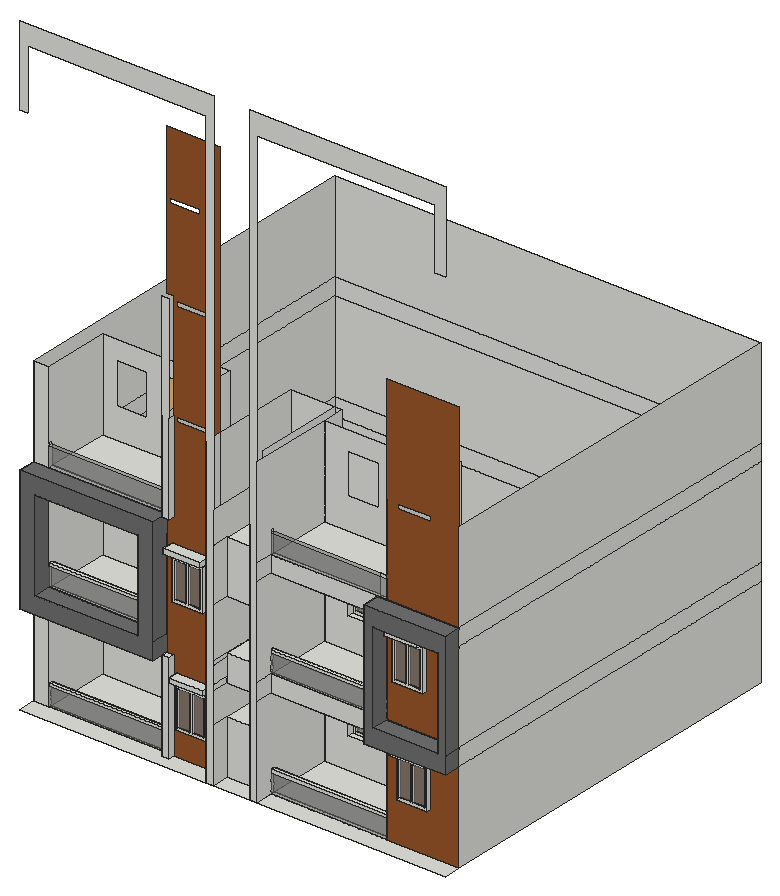
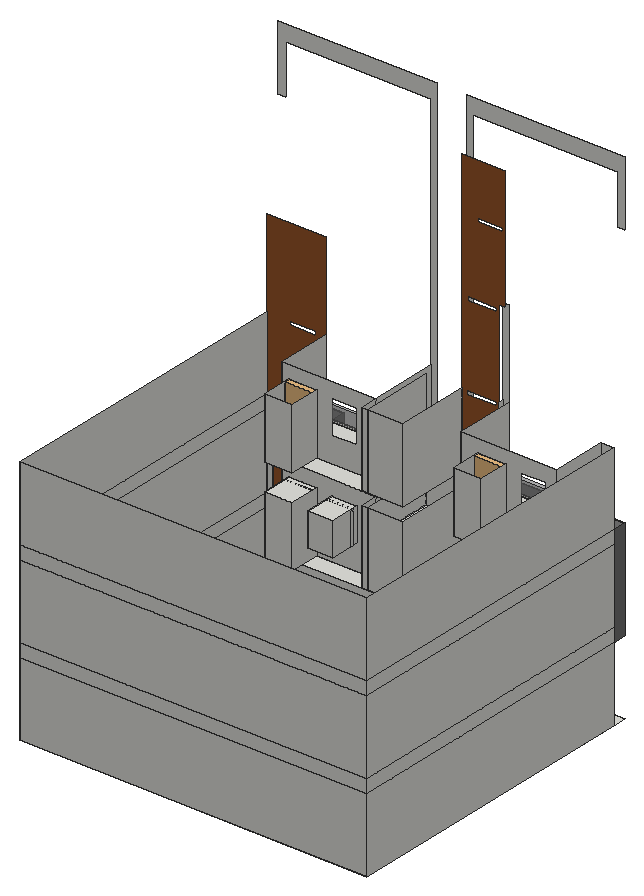
# SketchUp Ruby script. Lengths in inches.
U = 1.inch
M = Sketchup.active_model
def pt(a) = Geom::Point3d.new(a.map { |v| v * U })
def face(e, loops, mat)
  f = e.add_face(loops[0].map { |a| pt(a) })
  loops[1..].each { |l| e.add_face(l.map { |a| pt(a) }).erase! }
  f.material = f.back_material = mat if mat
  f
end
# faces: each face lists its corners as indices into pts; further lists are holes
def faces(e, pts, list, mat = nil) = list.each { |f| face(e, (f[0].is_a?(Array) ? f : [f]).map { |l| l.map { |i| pts[i] } }, mat) }
# xy, xz, yz: faces in a plane at the given z, y or x. An outline is a flat list of corners, or four numbers for a rectangle; further outlines are holes
def ring(l) = l.size == 4 ? [[l[0], l[1]], [l[2], l[1]], [l[2], l[3]], [l[0], l[3]]] : l.each_slice(2).to_a
def flat(e, list, mat, &to3) = list.each { |f| face(e, (f[0].is_a?(Array) ? f : [f]).map { |l| ring(l).map { |u, v| to3.(u, v) } }, mat) }
def xy(e, z, list, mat = nil) = flat(e, list, mat) { |x, y| [x, y, z] }
def xz(e, y, list, mat = nil) = flat(e, list, mat) { |x, z| [x, y, z] }
def yz(e, x, list, mat = nil) = flat(e, list, mat) { |y, z| [x, y, z] }
def lines(e, pts, list) = list.each { |a, b| e.add_line(pt(pts[a]), pt(pts[b])) }
# prism: a flat outline (further loops are holes) pulled along v
def prism(e, loops, v, mat = nil)
  f = face(e, loops, mat); d = Geom::Vector3d.new(v.map { |x| x * U })
  f.pushpull(f.normal.samedirection?(d) ? d.length : -d.length)
end
def box(e, o, s, mat = nil) = prism(e, [[o, [o[0] + s[0], o[1], o[2]], [o[0] + s[0], o[1] + s[1], o[2]], [o[0], o[1] + s[1], o[2]]]], [0, 0, s[2]], mat)
def at(x, y, z, deg = 0) = Geom::Transformation.translation(pt([x, y, z])) * Geom::Transformation.rotation(ORIGIN, Z_AXIS, deg.degrees)
def axes(o, x, y, z) = Geom::Transformation.new([*x, 0, *y, 0, *z, 0, *pt(o).to_a, 1])
def part(name) = M.definitions.add(name)
# library, detail: a bought-in or finely detailed component or shape, given as its bounding box
def library(name, o, s) = part(name).tap { |d| box(d.entities, o, s) }
def detail(e, o, s) = box(e.add_group.entities, o, s)
def put(e, d, t, mat = nil) = e.add_instance(d, t).tap { |i| i.material = mat if mat }
def group(e, t, mat = nil) = e.add_group.tap { |g| g.transformation = t; g.material = mat if mat }.entities
root = M.entities
M.materials.add("Generic").color = [112, 112, 112]
M.materials.add("[Translucent Glass Gray]").color = [128, 128, 128]
M.materials["[Translucent Glass Gray]"].alpha = 0.5
M.materials.add("[Wood Cherry Original]").color = [152, 86, 42]
c1 = library("Group\#1",[0,0,0],[54.125,10.375,118.625])
c2 = part("Group\#2")
xy(c2.entities,0,[[0,0,49,5]])
xy(c2.entities,4.23,[[4.23,0,22.39,2],[26.61,0,44.77,2]])
xy(c2.entities,60.71,[[4.23,0,22.39,2],[26.61,0,44.77,2]])
xy(c2.entities,64.9375,[[0,0,49,5]])
xz(c2.entities,0,[[[0,0,49,64.9375],[26.61,4.23,44.77,60.71],[4.23,4.23,22.39,60.71]]])
xz(c2.entities,2,[[4.23,4.23,22.39,60.71],[26.61,4.23,44.77,60.71]],"[Translucent Glass Gray]")
xz(c2.entities,5,[[0,0,49,64.9375]],"[Translucent Glass Gray]")
yz(c2.entities,0,[[0,0,5,64.9375]])
yz(c2.entities,4.23,[[0,4.23,2,60.71]])
yz(c2.entities,22.39,[[0,4.23,2,60.71]])
yz(c2.entities,26.61,[[0,4.23,2,60.71]])
yz(c2.entities,44.77,[[0,4.23,2,60.71]])
yz(c2.entities,49,[[0,0,5,64.9375]])
xy(root,170.875,[[0,79.8125,295.66,79.8125,295.66,106.875,223.17,106.875,223.17,97.1875,211.17,97.1875,211.17,106.875,0,106.875],[295.66,79.8125,295.66,249.5625,364.97,249.5625,364.97,106.875,307.66,106.875,307.66,79.8125],[307.66,79.8125,364.97,106.875],[364.97,79.8125,376.97,249.5625],[376.97,79.8125,676.6875,106.875],
  [211.17,97.1875,211.17,213.8125,178.54,213.8125,178.54,273.4375,124.42,273.4375,124.42,213.8125,24,213.8125,24,106.875,0,106.875,0,706.875,676.6875,706.875,676.6875,106.875,561.52,106.875,561.52,213.8125,546.92,213.8125,546.92,273.4375,492.79,273.4375,492.79,213.8125,376.97,213.8125,376.97,249.5625,295.66,249.5625,295.66,106.875,223.17,106.875,223.17,97.1875],[24,106.875,211.17,111.3125],[376.97,106.875,561.52,114.25],[24,111.3125,24,213.8125,124.42,213.8125,124.42,273.4375,178.54,273.4375,178.54,213.8125,211.17,213.8125,211.17,111.3125],[376.97,114.25,376.97,213.8125,492.79,213.8125,492.79,273.4375,546.92,273.4375,546.92,213.8125,561.52,213.8125,561.52,114.25]])
xy(root,201.375,[[24,106.875,211.17,111.3125],[376.97,106.875,561.52,114.25]])
xy(root,206.25,[[24,106.875,211.17,111.3125],[376.97,106.875,561.52,114.25]])
xy(root,220.08,[[46.11,213.8125,95.11,273.4375],[414.49,213.8125,463.49,273.4375]])
xy(root,257,[[307.66,106.875,364.97,195.8125]])
xy(root,284.05,[[228.07,91.5,282.2,106.875]])
xy(root,285.02,[[46.11,213.8125,95.11,273.4375],[414.49,213.8125,463.49,273.4375]])
xy(root,289.5,[[124.42,213.8125,178.54,273.4375],[492.79,213.8125,546.92,273.4375]])
xy(root,291.74,[[228.07,91.5,282.2,106.875]])
xy(root,303.3125,[[576.05,91.3125,633.05,106.875]])
xy(root,305.1875,[[307.66,106.875,364.97,195.8125]])
xy(root,311,[[576.05,91.3125,633.05,106.875]])
xy(root,314.875,[[211.17,97.1875,223.17,106.875],[24,106.875,211.17,213.8125],[376.97,106.875,561.52,213.8125]])
xy(root,314.875,[[0,79.8125,211.17,106.875],[547.21,79.8125,676.6875,106.875]],"Generic")
xy(root,341.75,[[187.3,106.875,187.3,112.6875,24,112.6875,24,213.8125,124.42,213.8125,124.42,273.4375,178.54,273.4375,178.54,213.8125,211.17,213.8125,211.17,106.875],[24,106.875,187.3,112.6875],[376.97,106.875,561.52,112.1875],[376.97,112.1875,376.97,213.8125,492.79,213.8125,492.79,273.4375,546.92,273.4375,546.92,213.8125,561.52,213.8125,561.52,112.1875]])
xy(root,341.75,[[24,79.8125,187.3,106.875],[561.52,79.8125,664.6875,106.875]],"Generic")
xy(root,348.375,[[307.66,106.875,364.97,195.8125]])
xy(root,372.25,[[24,106.875,187.3,112.6875],[376.97,106.875,561.52,112.1875]])
xy(root,377.125,[[24,106.875,187.3,112.6875],[376.97,106.875,561.52,112.1875]])
xy(root,390.96,[[46.11,213.8125,95.11,273.4375],[414.49,213.8125,463.49,273.4375]])
xy(root,428.625,[[307.66,106.875,364.97,195.8125]])
xy(root,455.9,[[46.11,213.8125,95.11,273.4375],[414.49,213.8125,463.49,273.4375]])
xy(root,460.375,[[124.42,213.8125,178.54,273.4375],[492.79,213.8125,546.92,273.4375]])
xy(root,466.99,[[220.82,88.0625,279.76,106.875]])
xy(root,471.77,[[570.12,91.3125,621.81,106.875]])
xy(root,474.67,[[220.82,88.0625,279.76,106.875]])
xy(root,479.46,[[570.12,91.3125,621.81,106.875]])
xy(root,485.75,[[24,79.8125,187.3,106.875],[24,106.875,211.17,213.8125],[376.97,106.875,561.52,213.8125]])
xy(root,485.75,[[561.52,79.8125,664.6875,106.875]],"Generic")
xy(root,512.625,[[211.17,97.1875,223.17,106.875],[24,106.875,211.17,113.625],[307.66,106.875,364.97,195.8125],[376.97,106.875,561.52,112.75],[376.97,112.75,376.97,213.8125,492.79,213.8125,492.79,273.4375,546.92,273.4375,546.92,213.8125,561.52,213.8125,561.52,112.75],
  [24,113.625,24,213.8125,124.42,213.8125,124.42,273.4375,178.54,273.4375,178.54,213.8125,211.17,213.8125,211.17,113.625]])
xy(root,512.625,[[0,79.8125,211.17,106.875],[547.21,79.8125,676.6875,106.875]],"Generic")
xz(root,79.8125,[[295.66,170.875,307.66,170.875,307.66,1153.3125,0,1153.3125,0,1025.25,12,1025.25,12,1121.625,295.66,1121.625],[364.97,170.875,376.97,170.875,376.97,1121.625,659.375,1121.625,659.375,1025.25,676.6875,1025.25,676.6875,1153.3125,364.97,1153.3125]])
xz(root,79.8125,[[[0,314.875,211.17,512.625],[24,341.75,187.3,485.75]],[[547.21,314.875,676.6875,512.625],[561.52,341.75,664.6875,485.75]]],"Generic")
xz(root,88.0625,[[220.82,466.99,279.76,474.67]])
xz(root,91.3125,[[576.05,303.3125,633.05,311],[570.12,471.77,621.81,479.46]])
xz(root,91.5,[[228.07,284.05,282.2,291.74]])
xz(root,97.1875,[[211.17,170.875,223.17,314.875],[211.17,512.625,223.17,827.5]])
xz(root,106.875,[[0,170.875,24,314.875],[307.66,170.875,364.97,257],[24,201.375,211.17,206.25],[376.97,201.375,561.52,206.25],[307.66,305.1875,364.97,348.375],
  [0,314.875,211.17,341.75],[376.97,314.875,547.21,341.75],[547.21,314.875,676.6875,341.75],[0,341.75,24,485.75],[187.3,341.75,211.17,485.75],
  [547.21,341.75,561.52,372.25],[664.6875,341.75,676.6875,485.75],[24,372.25,187.3,377.125],[376.97,372.25,547.21,377.125],[547.21,372.25,561.52,377.125],
  [547.21,377.125,561.52,485.75],[307.66,428.625,364.97,512.625],[0,485.75,211.17,512.625],[376.97,485.75,547.21,512.625],[547.21,485.75,676.6875,512.625],
  [0,512.625,24,656.625]])
xz(root,106.875,[[24,170.875,211.17,201.375],[376.97,170.875,561.52,201.375],[24,341.75,187.3,372.25],[376.97,341.75,547.21,372.25],[24,512.625,211.17,543.125],
  [376.97,512.625,561.52,543.125]],"[Translucent Glass Gray]")
xz(root,106.875,[[[223.17,170.875,295.66,170.875,295.66,1065.0625,211.17,1065.0625,211.17,827.5,223.17,827.5,223.17,512.625,211.17,512.625,211.17,314.875,223.17,314.875],[220.82,466.99,279.76,474.67],[228.07,648.74,285.2,656.42],[228.07,813.67,283.64,821.36],[228.07,284.05,282.2,291.74],[216.02,957.51,264.46,964.95]],[[561.52,170.875,676.6875,314.875],[576.05,303.3125,633.05,311]],[[561.52,341.75,664.6875,485.75],[570.12,471.77,621.81,479.46]],[[561.52,512.625,676.6875,827.5],[579.7,648.74,631.39,656.42]]],"[Wood Cherry Original]")
xz(root,111.3125,[[24,201.375,211.17,206.25]])
xz(root,111.3125,[[24,170.875,211.17,201.375]],"[Translucent Glass Gray]")
xz(root,112.1875,[[547.21,341.75,561.52,372.25],[376.97,372.25,547.21,377.125],[547.21,372.25,561.52,377.125]])
xz(root,112.1875,[[376.97,341.75,547.21,372.25]],"[Translucent Glass Gray]")
xz(root,112.6875,[[24,372.25,187.3,377.125]])
xz(root,112.6875,[[24,341.75,187.3,372.25]],"[Translucent Glass Gray]")
xz(root,112.75,[[547.21,512.625,561.52,543.125]])
xz(root,112.75,[[376.97,512.625,547.21,543.125]],"[Translucent Glass Gray]")
xz(root,113.625,[[24,512.625,211.17,543.125]],"[Translucent Glass Gray]")
xz(root,114.25,[[376.97,201.375,561.52,206.25]])
xz(root,114.25,[[376.97,170.875,561.52,201.375]],"[Translucent Glass Gray]")
xz(root,195.8125,[[307.66,257,364.97,305.1875],[307.66,305.1875,364.97,314.875],[307.66,341.75,364.97,348.375],[307.66,348.375,364.97,428.625],[307.66,512.625,364.97,563.98]])
xz(root,213.8125,[[[24,170.875,124.42,170.875,124.42,289.5,178.54,289.5,178.54,170.875,211.17,170.875,211.17,314.875,24,314.875],[46.11,220.08,95.11,285.02]],[[376.97,170.875,492.79,170.875,492.79,289.5,546.92,289.5,546.92,170.875,561.52,170.875,561.52,314.875,376.97,314.875],[414.49,220.08,463.49,285.02]],[[24,341.75,124.42,341.75,124.42,460.375,178.54,460.375,178.54,341.75,211.17,341.75,211.17,485.75,24,485.75],[46.11,390.96,95.11,455.9]],[[376.97,341.75,492.79,341.75,492.79,460.375,546.92,460.375,546.92,341.75,561.52,341.75,561.52,485.75,376.97,485.75],[414.49,390.96,463.49,455.9]],[[24,512.625,124.42,512.625,124.42,631.25,178.54,631.25,178.54,512.625,211.17,512.625,211.17,656.625,24,656.625],[46.11,561.83,95.11,626.77]],
  [[376.97,512.625,492.79,512.625,492.79,631.25,546.92,631.25,546.92,512.625,561.52,512.625,561.52,656.625,376.97,656.625],[414.49,561.83,463.49,626.77]]])
xz(root,249.5625,[[295.66,170.875,364.97,314.875],[364.97,170.875,376.97,314.875],[295.66,341.75,364.97,485.75],[364.97,341.75,376.97,485.75],[295.66,512.625,364.97,656.625],
  [364.97,512.625,376.97,656.625]])
xz(root,273.4375,[[124.42,170.875,178.54,289.5],[492.79,170.875,546.92,289.5],[46.11,220.08,95.11,285.02],[414.49,220.08,463.49,285.02],[124.42,341.75,178.54,460.375],
  [492.79,341.75,546.92,460.375],[46.11,390.96,95.11,455.9],[414.49,390.96,463.49,455.9],[124.42,512.625,178.54,631.25],[492.79,512.625,546.92,631.25]])
xz(root,706.875,[[0,170.875,676.6875,314.875],[0,314.875,676.6875,341.75],[0,341.75,676.6875,485.75],[0,485.75,676.6875,512.625],[0,512.625,676.6875,656.625]])
yz(root,0,[[106.875,170.875,706.875,314.875],[106.875,314.875,706.875,341.75],[106.875,341.75,706.875,485.75],[106.875,485.75,706.875,512.625],[106.875,512.625,706.875,656.625]])
yz(root,0,[[79.8125,314.875,106.875,512.625]],"Generic")
yz(root,24,[[106.875,170.875,111.3125,201.375],[111.3125,170.875,213.8125,170.875,213.8125,314.875,106.875,314.875,106.875,206.25,111.3125,206.25],[106.875,201.375,111.3125,206.25],[106.875,341.75,112.6875,372.25],[112.6875,341.75,213.8125,341.75,213.8125,485.75,106.875,485.75,106.875,377.125,112.6875,377.125],
  [106.875,372.25,112.6875,377.125],[106.875,512.625,113.625,543.125],[113.625,512.625,213.8125,512.625,213.8125,656.625,106.875,656.625,106.875,548,113.625,548]])
yz(root,24,[[79.8125,341.75,106.875,485.75]],"Generic")
yz(root,46.11,[[213.8125,220.08,273.4375,285.02],[213.8125,390.96,273.4375,455.9]])
yz(root,95.11,[[213.8125,220.08,273.4375,285.02],[213.8125,390.96,273.4375,455.9]])
yz(root,124.42,[[213.8125,170.875,273.4375,289.5],[213.8125,341.75,273.4375,460.375],[213.8125,512.625,273.4375,631.25]])
yz(root,178.54,[[213.8125,170.875,273.4375,289.5],[213.8125,341.75,273.4375,460.375],[213.8125,512.625,273.4375,631.25]])
yz(root,187.3,[[106.875,341.75,112.6875,372.25],[106.875,372.25,112.6875,377.125]])
yz(root,187.3,[[79.8125,341.75,106.875,485.75]],"Generic")
yz(root,211.17,[[97.1875,170.875,97.1875,314.875,213.8125,314.875,213.8125,170.875,111.3125,170.875,111.3125,206.25,106.875,206.25,106.875,170.875],[106.875,170.875,111.3125,201.375],[106.875,201.375,111.3125,206.25],[106.875,341.75,213.8125,485.75],[97.1875,512.625,97.1875,656.625,213.8125,656.625,213.8125,512.625,113.625,512.625,113.625,548,106.875,548,106.875,512.625],
  [106.875,512.625,113.625,543.125]])
yz(root,211.17,[[79.8125,314.875,106.875,341.75],[79.8125,341.75,106.875,512.625]],"Generic")
yz(root,220.82,[[88.0625,466.99,106.875,474.67]])
yz(root,223.17,[[97.1875,170.875,106.875,314.875],[97.1875,512.625,106.875,656.625]])
yz(root,228.07,[[91.5,284.05,106.875,291.74]])
yz(root,279.76,[[88.0625,466.99,106.875,474.67]])
yz(root,282.2,[[91.5,284.05,106.875,291.74]])
yz(root,295.66,[[79.8125,170.875,106.875,314.875],[106.875,170.875,249.5625,314.875],[79.8125,314.875,106.875,341.75],[79.8125,341.75,106.875,485.75],[106.875,341.75,249.5625,485.75],
  [79.8125,485.75,106.875,512.625],[79.8125,512.625,106.875,656.625],[106.875,512.625,249.5625,656.625]])
yz(root,307.66,[[79.8125,170.875,106.875,257],[79.8125,257,195.8125,305.1875],[79.8125,305.1875,106.875,314.875],[106.875,305.1875,195.8125,314.875],[79.8125,314.875,106.875,341.75],
  [79.8125,341.75,106.875,348.375],[106.875,341.75,195.8125,348.375],[79.8125,348.375,195.8125,428.625],[79.8125,428.625,106.875,512.625],[79.8125,512.625,195.8125,563.98]])
yz(root,364.97,[[79.8125,170.875,106.875,257],[106.875,170.875,106.875,257,195.8125,257,195.8125,314.875,249.5625,314.875,249.5625,170.875],[79.8125,257,195.8125,305.1875],[79.8125,305.1875,106.875,314.875],[106.875,305.1875,195.8125,314.875],
  [79.8125,314.875,106.875,341.75],[79.8125,341.75,106.875,348.375],[106.875,341.75,195.8125,348.375],[195.8125,341.75,195.8125,428.625,106.875,428.625,106.875,485.75,249.5625,485.75,249.5625,341.75],[79.8125,348.375,195.8125,428.625],
  [79.8125,428.625,106.875,485.75],[79.8125,485.75,106.875,512.625],[79.8125,512.625,195.8125,563.98],[195.8125,512.625,195.8125,563.98,106.875,563.98,106.875,656.625,249.5625,656.625,249.5625,512.625]])
yz(root,376.97,[[79.8125,170.875,106.875,170.875,106.875,206.25,114.25,206.25,114.25,170.875,213.8125,170.875,213.8125,314.875,79.8125,314.875],[106.875,170.875,114.25,201.375],[213.8125,170.875,249.5625,314.875],[106.875,201.375,114.25,206.25],[79.8125,314.875,106.875,341.75],
  [79.8125,341.75,106.875,341.75,106.875,377.125,112.1875,377.125,112.1875,341.75,213.8125,341.75,213.8125,485.75,79.8125,485.75],[106.875,341.75,112.1875,372.25],[213.8125,341.75,249.5625,485.75],[106.875,372.25,112.1875,377.125],[79.8125,485.75,106.875,512.625],
  [79.8125,512.625,106.875,512.625,106.875,548,112.75,548,112.75,512.625,213.8125,512.625,213.8125,656.625,79.8125,656.625],[106.875,512.625,112.75,543.125],[213.8125,512.625,249.5625,656.625]])
yz(root,414.49,[[213.8125,220.08,273.4375,285.02],[213.8125,390.96,273.4375,455.9]])
yz(root,463.49,[[213.8125,220.08,273.4375,285.02],[213.8125,390.96,273.4375,455.9]])
yz(root,492.79,[[213.8125,170.875,273.4375,289.5],[213.8125,341.75,273.4375,460.375],[213.8125,512.625,273.4375,631.25]])
yz(root,546.92,[[213.8125,170.875,273.4375,289.5],[213.8125,341.75,273.4375,460.375],[213.8125,512.625,273.4375,631.25]])
yz(root,547.21,[[79.8125,314.875,106.875,512.625]],"Generic")
yz(root,561.52,[[106.875,170.875,114.25,201.375],[114.25,170.875,114.25,206.25,106.875,206.25,106.875,314.875,213.8125,314.875,213.8125,170.875],[106.875,201.375,114.25,206.25],[106.875,341.75,112.1875,372.25],[112.1875,341.75,112.1875,377.125,106.875,377.125,106.875,485.75,213.8125,485.75,213.8125,341.75],
  [106.875,372.25,112.1875,377.125],[106.875,512.625,112.75,543.125],[112.75,512.625,112.75,548,106.875,548,106.875,656.625,213.8125,656.625,213.8125,512.625]])
yz(root,561.52,[[79.8125,341.75,106.875,485.75]],"Generic")
yz(root,570.12,[[91.3125,471.77,106.875,479.46]])
yz(root,576.05,[[91.3125,303.3125,106.875,311]])
yz(root,621.81,[[91.3125,471.77,106.875,479.46]])
yz(root,633.05,[[91.3125,303.3125,106.875,311]])
yz(root,664.6875,[[79.8125,341.75,106.875,485.75]],"Generic")
yz(root,676.6875,[[106.875,170.875,706.875,314.875],[106.875,314.875,706.875,341.75],[106.875,341.75,706.875,485.75],[106.875,485.75,706.875,512.625],[106.875,512.625,706.875,656.625]])
yz(root,676.6875,[[79.8125,314.875,106.875,341.75],[79.8125,341.75,106.875,512.625]],"Generic")
put(root,c1,at(492.79,213.8125,170.875))
put(root,c1,at(124.42,213.8125,170.875))
put(root,c2,at(229.91,101.875,212.71))
put(root,c2,at(414.49,224.0625,218.71))
put(root,c2,at(46.11,224.0625,218.71))
put(root,c2,at(581.29,101.875,237.14))
put(root,c1,at(492.79,213.8125,341.75))
put(root,c1,at(124.42,213.8125,341.75))
put(root,c2,at(46.11,224.0625,389.58))
put(root,c2,at(414.49,224.0625,390.96))
put(root,c2,at(224.11,101.875,394.07))
put(root,c2,at(574.46,101.875,403.01))
put(root,c1,at(492.79,213.8125,512.625))
put(root,c1,at(124.42,213.8125,512.625))
